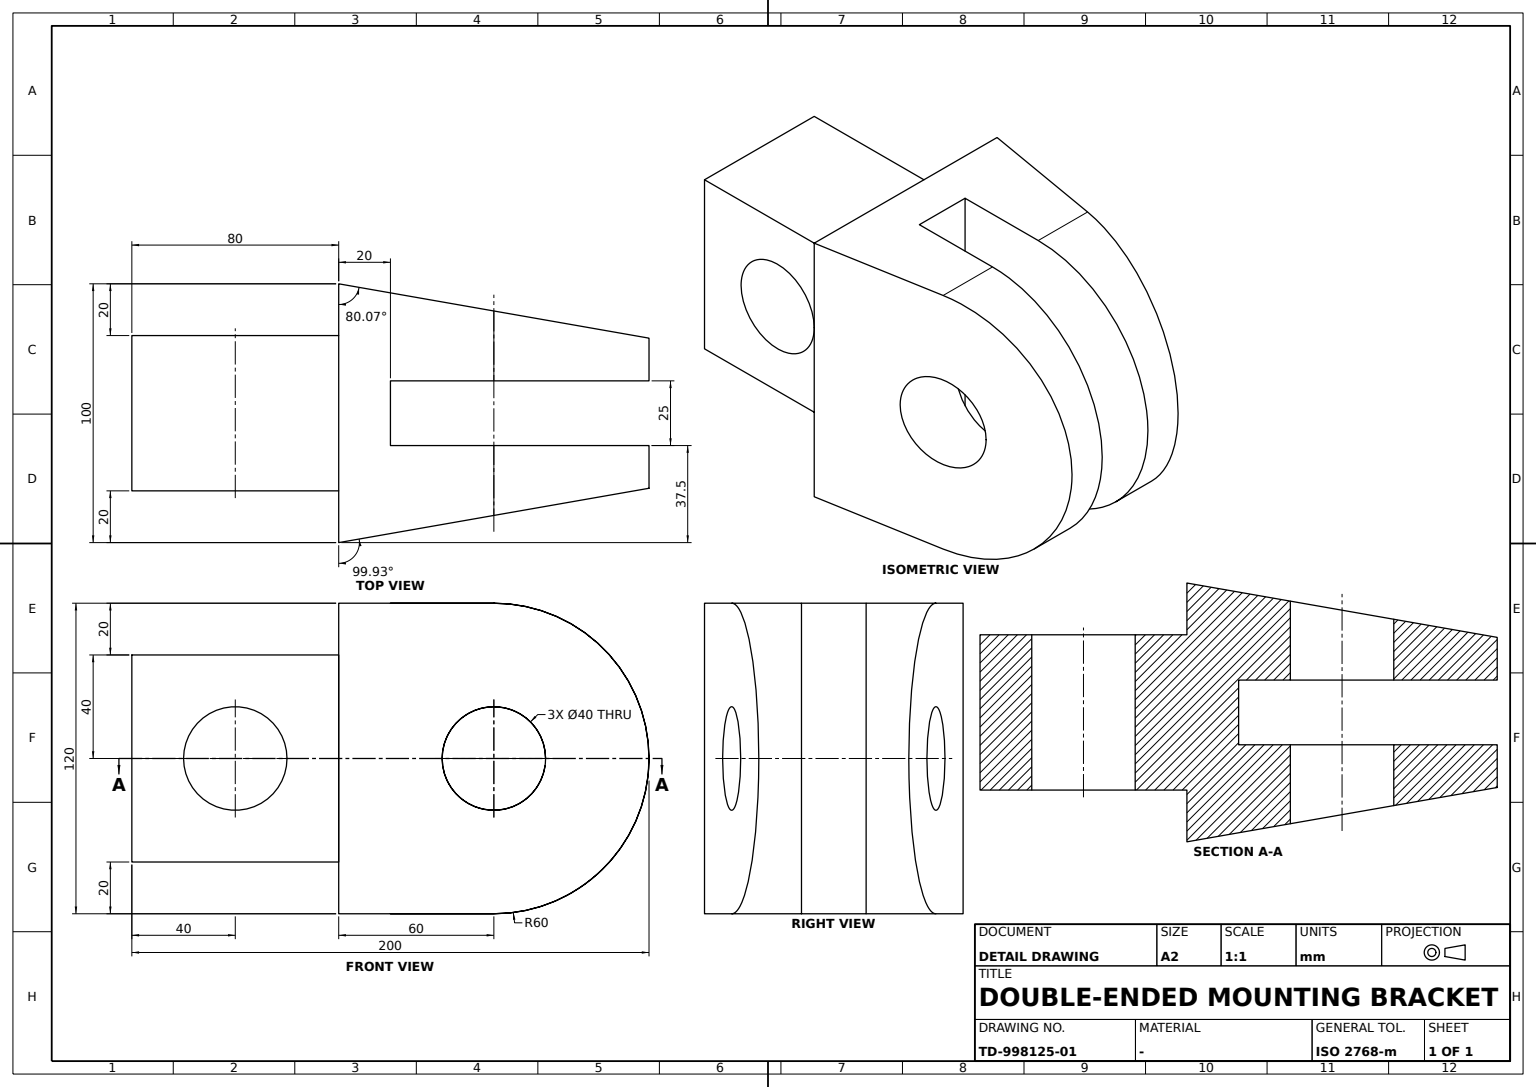
ISO-10303-21;
HEADER;
FILE_DESCRIPTION((''),'2;1');
FILE_NAME('','',(''),(''),'','','');
FILE_SCHEMA(('AUTOMOTIVE_DESIGN'));
ENDSEC;
DATA;
#1=APPLICATION_CONTEXT('');
#2=PRODUCT_CONTEXT('',#1,'mechanical');
#3=PRODUCT('','','',(#2));
#4=PRODUCT_DEFINITION_FORMATION('','',#3);
#5=PRODUCT_DEFINITION_CONTEXT('',#1,'design');
#6=PRODUCT_DEFINITION('','',#4,#5);
#7=PRODUCT_DEFINITION_SHAPE('','',#6);
#8=(LENGTH_UNIT()NAMED_UNIT(*)SI_UNIT(.MILLI.,.METRE.));
#9=(NAMED_UNIT(*)PLANE_ANGLE_UNIT()SI_UNIT($,.RADIAN.));
#10=(NAMED_UNIT(*)SI_UNIT($,.STERADIAN.)SOLID_ANGLE_UNIT());
#11=UNCERTAINTY_MEASURE_WITH_UNIT(LENGTH_MEASURE(1.E-05),#8,'distance_accuracy_value','');
#12=(GEOMETRIC_REPRESENTATION_CONTEXT(3)GLOBAL_UNCERTAINTY_ASSIGNED_CONTEXT((#11))GLOBAL_UNIT_ASSIGNED_CONTEXT((#8,#9,#10))REPRESENTATION_CONTEXT('',''));
#13=CARTESIAN_POINT('',(12.5,-40.,-60.));
#14=VERTEX_POINT('',#13);
#15=CARTESIAN_POINT('',(12.5,0.,-60.));
#16=VERTEX_POINT('',#15);
#17=CARTESIAN_POINT('',(12.5,-20.,-60.));
#18=DIRECTION('',(0.,1.,0.));
#19=VECTOR('',#18,1000.);
#20=LINE('',#17,#19);
#21=EDGE_CURVE('',#14,#16,#20,.T.);
#22=ORIENTED_EDGE('',*,*,#21,.F.);
#23=CARTESIAN_POINT('',(12.5,-40.,60.));
#24=VERTEX_POINT('',#23);
#25=CARTESIAN_POINT('',(12.5,-40.,0.));
#26=DIRECTION('',(0.,0.,-1.));
#27=VECTOR('',#26,1000.);
#28=LINE('',#25,#27);
#29=EDGE_CURVE('',#24,#14,#28,.T.);
#30=ORIENTED_EDGE('',*,*,#29,.F.);
#31=CARTESIAN_POINT('',(12.5,0.,60.));
#32=VERTEX_POINT('',#31);
#33=CARTESIAN_POINT('',(12.5,-20.,60.));
#34=LINE('',#33,#19);
#35=EDGE_CURVE('',#24,#32,#34,.T.);
#36=ORIENTED_EDGE('',*,*,#35,.T.);
#37=CARTESIAN_POINT('',(12.5,60.,0.));
#38=VERTEX_POINT('',#37);
#39=CARTESIAN_POINT('',(12.5,0.,0.));
#40=DIRECTION('',(1.,0.,0.));
#41=DIRECTION('',(0.,-1.,0.));
#42=AXIS2_PLACEMENT_3D('',#39,#40,#41);
#43=CIRCLE('',#42,60.);
#44=EDGE_CURVE('',#38,#32,#43,.T.);
#45=ORIENTED_EDGE('',*,*,#44,.F.);
#46=EDGE_CURVE('',#16,#38,#43,.T.);
#47=ORIENTED_EDGE('',*,*,#46,.F.);
#48=EDGE_LOOP('',(#22,#30,#36,#45,#47));
#49=FACE_OUTER_BOUND('',#48,.T.);
#50=CARTESIAN_POINT('',(12.5,20.,0.));
#51=VERTEX_POINT('',#50);
#52=CARTESIAN_POINT('',(12.5,-20.,0.));
#53=VERTEX_POINT('',#52);
#54=CIRCLE('',#42,20.);
#55=EDGE_CURVE('',#51,#53,#54,.T.);
#56=ORIENTED_EDGE('',*,*,#55,.T.);
#57=EDGE_CURVE('',#53,#51,#54,.T.);
#58=ORIENTED_EDGE('',*,*,#57,.T.);
#59=EDGE_LOOP('',(#56,#58));
#60=FACE_BOUND('',#59,.T.);
#61=CARTESIAN_POINT('',(12.5,77.214676,60.));
#62=AXIS2_PLACEMENT_3D('',#61,#40,#41);
#63=PLANE('',#62);
#64=ADVANCED_FACE('',(#49,#60),#63,.F.);
#65=CARTESIAN_POINT('',(-12.5,20.,0.));
#66=VERTEX_POINT('',#65);
#67=CARTESIAN_POINT('',(-12.5,-20.,0.));
#68=VERTEX_POINT('',#67);
#69=CARTESIAN_POINT('',(-12.5,0.,0.));
#70=DIRECTION('',(-1.,0.,0.));
#71=AXIS2_PLACEMENT_3D('',#69,#70,#18);
#72=CIRCLE('',#71,20.);
#73=EDGE_CURVE('',#66,#68,#72,.T.);
#74=ORIENTED_EDGE('',*,*,#73,.F.);
#75=CARTESIAN_POINT('',(-36.,20.,0.));
#76=VERTEX_POINT('',#75);
#77=CARTESIAN_POINT('',(-0.66,20.,0.));
#78=VECTOR('',#70,1000.);
#79=LINE('',#77,#78);
#80=EDGE_CURVE('',#66,#76,#79,.T.);
#81=ORIENTED_EDGE('',*,*,#80,.T.);
#82=CARTESIAN_POINT('',(-42.999999,-20.,0.));
#83=VERTEX_POINT('',#82);
#84=CARTESIAN_POINT('',(-42.999999,-19.999994,-1.218732));
#85=CARTESIAN_POINT('',(-42.983753,-19.90716,-2.437462));
#86=CARTESIAN_POINT('',(-42.951263,-19.721501,-3.646476));
#87=CARTESIAN_POINT('',(-42.833603,-19.049161,-6.535238));
#88=CARTESIAN_POINT('',(-42.625053,-17.857447,-9.25575));
#89=CARTESIAN_POINT('',(-42.472523,-16.985847,-10.771201));
#90=CARTESIAN_POINT('',(-42.11097,-14.919828,-13.601309));
#91=CARTESIAN_POINT('',(-41.652871,-12.30212,-15.914277));
#92=CARTESIAN_POINT('',(-41.401497,-10.865696,-16.926953));
#93=CARTESIAN_POINT('',(-40.839949,-7.656852,-18.700547));
#94=CARTESIAN_POINT('',(-40.223795,-4.135971,-19.70666));
#95=CARTESIAN_POINT('',(-39.892721,-2.24412,-20.010333));
#96=CARTESIAN_POINT('',(-39.250249,1.427151,-20.157864));
#97=CARTESIAN_POINT('',(-38.618783,5.035523,-19.47528));
#98=CARTESIAN_POINT('',(-38.322943,6.726041,-18.958274));
#99=CARTESIAN_POINT('',(-37.757941,9.954625,-17.566907));
#100=CARTESIAN_POINT('',(-37.257588,12.813783,-15.505126));
#101=CARTESIAN_POINT('',(-37.028803,14.121128,-14.325447));
#102=CARTESIAN_POINT('',(-36.621836,16.446649,-11.710301));
#103=CARTESIAN_POINT('',(-36.32202,18.159888,-8.646962));
#104=CARTESIAN_POINT('',(-36.202412,18.84336,-7.035318));
#105=CARTESIAN_POINT('',(-36.077188,19.558925,-4.653904));
#106=CARTESIAN_POINT('',(-36.01769,19.898913,-2.200641));
#107=CARTESIAN_POINT('',(-36.005897,19.966304,-1.468511));
#108=CARTESIAN_POINT('',(-36.,20.,-0.734255));
#109=B_SPLINE_CURVE_WITH_KNOTS('',5,(#82,#84,#85,#86,#87,#88,#89,#90,#91,#92,#93,#94,#95,#96,#97,#98,#99,#100,#101,#102,#103,#104,#105,#106,#107,#108,#75),.UNSPECIFIED.,.F.,.F.,(6,3,3,3,3,3,3,3,6),(89.533426243,98.151203404,110.460544169,122.915174615,136.537729583,149.11185729,161.567661291,173.874806578,179.066776811),.UNSPECIFIED.);
#110=EDGE_CURVE('',#83,#76,#109,.T.);
#111=ORIENTED_EDGE('',*,*,#110,.F.);
#112=CARTESIAN_POINT('',(-0.66,-20.,0.));
#113=LINE('',#112,#78);
#114=EDGE_CURVE('',#68,#83,#113,.T.);
#115=ORIENTED_EDGE('',*,*,#114,.F.);
#116=EDGE_LOOP('',(#74,#81,#111,#115));
#117=FACE_OUTER_BOUND('',#116,.T.);
#118=CARTESIAN_POINT('',(-0.66,0.,0.));
#119=AXIS2_PLACEMENT_3D('',#118,#70,#18);
#120=CYLINDRICAL_SURFACE('',#119,20.);
#121=ADVANCED_FACE('',(#117),#120,.F.);
#122=CARTESIAN_POINT('',(-50.,-60.,60.));
#123=VERTEX_POINT('',#122);
#124=CARTESIAN_POINT('',(50.,-60.,60.));
#125=VERTEX_POINT('',#124);
#126=CARTESIAN_POINT('',(0.,-60.,60.));
#127=VECTOR('',#40,1000.);
#128=LINE('',#126,#127);
#129=EDGE_CURVE('',#123,#125,#128,.T.);
#130=ORIENTED_EDGE('',*,*,#129,.F.);
#131=CARTESIAN_POINT('',(-50.,-60.,-60.));
#132=VERTEX_POINT('',#131);
#133=CARTESIAN_POINT('',(-50.,-60.,0.));
#134=LINE('',#133,#27);
#135=EDGE_CURVE('',#123,#132,#134,.T.);
#136=ORIENTED_EDGE('',*,*,#135,.T.);
#137=CARTESIAN_POINT('',(50.,-60.,-60.));
#138=VERTEX_POINT('',#137);
#139=CARTESIAN_POINT('',(0.,-60.,-60.));
#140=LINE('',#139,#127);
#141=EDGE_CURVE('',#132,#138,#140,.T.);
#142=ORIENTED_EDGE('',*,*,#141,.T.);
#143=CARTESIAN_POINT('',(50.,-60.,0.));
#144=LINE('',#143,#27);
#145=EDGE_CURVE('',#125,#138,#144,.T.);
#146=ORIENTED_EDGE('',*,*,#145,.F.);
#147=EDGE_LOOP('',(#130,#136,#142,#146));
#148=FACE_OUTER_BOUND('',#147,.T.);
#149=CARTESIAN_POINT('',(30.,-60.,-40.));
#150=VERTEX_POINT('',#149);
#151=CARTESIAN_POINT('',(30.,-60.,40.));
#152=VERTEX_POINT('',#151);
#153=CARTESIAN_POINT('',(30.,-60.,0.));
#154=DIRECTION('',(0.,0.,1.));
#155=VECTOR('',#154,1000.);
#156=LINE('',#153,#155);
#157=EDGE_CURVE('',#150,#152,#156,.T.);
#158=ORIENTED_EDGE('',*,*,#157,.F.);
#159=CARTESIAN_POINT('',(-30.,-60.,-40.));
#160=VERTEX_POINT('',#159);
#161=CARTESIAN_POINT('',(0.,-60.,-40.));
#162=LINE('',#161,#127);
#163=EDGE_CURVE('',#160,#150,#162,.T.);
#164=ORIENTED_EDGE('',*,*,#163,.F.);
#165=CARTESIAN_POINT('',(-30.,-60.,40.));
#166=VERTEX_POINT('',#165);
#167=CARTESIAN_POINT('',(-30.,-60.,0.));
#168=LINE('',#167,#155);
#169=EDGE_CURVE('',#160,#166,#168,.T.);
#170=ORIENTED_EDGE('',*,*,#169,.T.);
#171=CARTESIAN_POINT('',(0.,-60.,40.));
#172=LINE('',#171,#127);
#173=EDGE_CURVE('',#166,#152,#172,.T.);
#174=ORIENTED_EDGE('',*,*,#173,.T.);
#175=EDGE_LOOP('',(#158,#164,#170,#174));
#176=FACE_BOUND('',#175,.T.);
#177=AXIS2_PLACEMENT_3D('',#126,#41,#26);
#178=PLANE('',#177);
#179=ADVANCED_FACE('',(#148,#176),#178,.T.);
#180=CARTESIAN_POINT('',(-30.,-140.,-40.));
#181=VERTEX_POINT('',#180);
#182=CARTESIAN_POINT('',(-30.,-100.,-40.));
#183=LINE('',#182,#19);
#184=EDGE_CURVE('',#181,#160,#183,.T.);
#185=ORIENTED_EDGE('',*,*,#184,.F.);
#186=CARTESIAN_POINT('',(-30.,-140.,40.));
#187=VERTEX_POINT('',#186);
#188=CARTESIAN_POINT('',(-30.,-140.,0.));
#189=LINE('',#188,#27);
#190=EDGE_CURVE('',#187,#181,#189,.T.);
#191=ORIENTED_EDGE('',*,*,#190,.F.);
#192=CARTESIAN_POINT('',(-30.,-100.,40.));
#193=VECTOR('',#41,1000.);
#194=LINE('',#192,#193);
#195=EDGE_CURVE('',#166,#187,#194,.T.);
#196=ORIENTED_EDGE('',*,*,#195,.F.);
#197=ORIENTED_EDGE('',*,*,#169,.F.);
#198=EDGE_LOOP('',(#185,#191,#196,#197));
#199=FACE_OUTER_BOUND('',#198,.T.);
#200=CARTESIAN_POINT('',(-30.,-80.,0.));
#201=VERTEX_POINT('',#200);
#202=CARTESIAN_POINT('',(-30.,-120.,0.));
#203=VERTEX_POINT('',#202);
#204=CARTESIAN_POINT('',(-30.,-100.,0.));
#205=AXIS2_PLACEMENT_3D('',#204,#40,#18);
#206=CIRCLE('',#205,20.);
#207=EDGE_CURVE('',#201,#203,#206,.T.);
#208=ORIENTED_EDGE('',*,*,#207,.T.);
#209=EDGE_CURVE('',#203,#201,#206,.T.);
#210=ORIENTED_EDGE('',*,*,#209,.T.);
#211=EDGE_LOOP('',(#208,#210));
#212=FACE_BOUND('',#211,.T.);
#213=CARTESIAN_POINT('',(-30.,0.,0.));
#214=AXIS2_PLACEMENT_3D('',#213,#40,#18);
#215=PLANE('',#214);
#216=ADVANCED_FACE('',(#199,#212),#215,.F.);
#217=CARTESIAN_POINT('',(30.,-120.,0.));
#218=VERTEX_POINT('',#217);
#219=CARTESIAN_POINT('',(-10.66,-120.,0.));
#220=LINE('',#219,#78);
#221=EDGE_CURVE('',#218,#203,#220,.T.);
#222=ORIENTED_EDGE('',*,*,#221,.F.);
#223=CARTESIAN_POINT('',(30.,-80.,0.));
#224=VERTEX_POINT('',#223);
#225=CARTESIAN_POINT('',(30.,-100.,0.));
#226=AXIS2_PLACEMENT_3D('',#225,#40,#18);
#227=CIRCLE('',#226,20.);
#228=EDGE_CURVE('',#218,#224,#227,.T.);
#229=ORIENTED_EDGE('',*,*,#228,.T.);
#230=CARTESIAN_POINT('',(-10.66,-80.,0.));
#231=LINE('',#230,#78);
#232=EDGE_CURVE('',#224,#201,#231,.T.);
#233=ORIENTED_EDGE('',*,*,#232,.T.);
#234=ORIENTED_EDGE('',*,*,#209,.F.);
#235=EDGE_LOOP('',(#222,#229,#233,#234));
#236=FACE_OUTER_BOUND('',#235,.T.);
#237=CARTESIAN_POINT('',(-10.66,-100.,0.));
#238=AXIS2_PLACEMENT_3D('',#237,#70,#18);
#239=CYLINDRICAL_SURFACE('',#238,20.);
#240=ADVANCED_FACE('',(#236),#239,.F.);
#241=CARTESIAN_POINT('',(30.,-140.,-40.));
#242=VERTEX_POINT('',#241);
#243=CARTESIAN_POINT('',(0.,-140.,-40.));
#244=LINE('',#243,#127);
#245=EDGE_CURVE('',#181,#242,#244,.T.);
#246=ORIENTED_EDGE('',*,*,#245,.F.);
#247=ORIENTED_EDGE('',*,*,#184,.T.);
#248=ORIENTED_EDGE('',*,*,#163,.T.);
#249=CARTESIAN_POINT('',(30.,-100.,-40.));
#250=LINE('',#249,#19);
#251=EDGE_CURVE('',#242,#150,#250,.T.);
#252=ORIENTED_EDGE('',*,*,#251,.F.);
#253=EDGE_LOOP('',(#246,#247,#248,#252));
#254=FACE_OUTER_BOUND('',#253,.T.);
#255=AXIS2_PLACEMENT_3D('',#243,#26,#18);
#256=PLANE('',#255);
#257=ADVANCED_FACE('',(#254),#256,.T.);
#258=ORIENTED_EDGE('',*,*,#73,.T.);
#259=EDGE_CURVE('',#68,#66,#72,.T.);
#260=ORIENTED_EDGE('',*,*,#259,.T.);
#261=EDGE_LOOP('',(#258,#260));
#262=FACE_BOUND('',#261,.T.);
#263=CARTESIAN_POINT('',(-12.5,0.,60.));
#264=VERTEX_POINT('',#263);
#265=CARTESIAN_POINT('',(-12.5,-40.,60.));
#266=VERTEX_POINT('',#265);
#267=CARTESIAN_POINT('',(-12.5,-20.,60.));
#268=LINE('',#267,#193);
#269=EDGE_CURVE('',#264,#266,#268,.T.);
#270=ORIENTED_EDGE('',*,*,#269,.T.);
#271=CARTESIAN_POINT('',(-12.5,-40.,-60.));
#272=VERTEX_POINT('',#271);
#273=CARTESIAN_POINT('',(-12.5,-40.,0.));
#274=LINE('',#273,#27);
#275=EDGE_CURVE('',#266,#272,#274,.T.);
#276=ORIENTED_EDGE('',*,*,#275,.T.);
#277=CARTESIAN_POINT('',(-12.5,0.,-60.));
#278=VERTEX_POINT('',#277);
#279=CARTESIAN_POINT('',(-12.5,-20.,-60.));
#280=LINE('',#279,#19);
#281=EDGE_CURVE('',#272,#278,#280,.T.);
#282=ORIENTED_EDGE('',*,*,#281,.T.);
#283=CARTESIAN_POINT('',(-12.5,60.,0.));
#284=VERTEX_POINT('',#283);
#285=CIRCLE('',#71,60.);
#286=EDGE_CURVE('',#284,#278,#285,.T.);
#287=ORIENTED_EDGE('',*,*,#286,.F.);
#288=EDGE_CURVE('',#264,#284,#285,.T.);
#289=ORIENTED_EDGE('',*,*,#288,.F.);
#290=EDGE_LOOP('',(#270,#276,#282,#287,#289));
#291=FACE_OUTER_BOUND('',#290,.T.);
#292=AXIS2_PLACEMENT_3D('',#265,#70,#18);
#293=PLANE('',#292);
#294=ADVANCED_FACE('',(#262,#291),#293,.F.);
#295=CARTESIAN_POINT('',(-39.5,0.,60.));
#296=VERTEX_POINT('',#295);
#297=CARTESIAN_POINT('',(-44.75,-30.,60.));
#298=DIRECTION('',(0.172380332,0.985030467,0.));
#299=VECTOR('',#298,1000.);
#300=LINE('',#297,#299);
#301=EDGE_CURVE('',#123,#296,#300,.T.);
#302=ORIENTED_EDGE('',*,*,#301,.T.);
#303=CARTESIAN_POINT('',(-29.,60.,0.));
#304=VERTEX_POINT('',#303);
#305=CARTESIAN_POINT('',(-29.,59.999999,3.493208));
#306=CARTESIAN_POINT('',(-29.044489,59.745776,6.986413));
#307=CARTESIAN_POINT('',(-29.133467,59.237334,10.454186));
#308=CARTESIAN_POINT('',(-29.437777,57.498419,18.28685));
#309=CARTESIAN_POINT('',(-29.964905,54.486256,25.726527));
#310=CARTESIAN_POINT('',(-30.329947,52.400304,29.744072));
#311=CARTESIAN_POINT('',(-31.190529,47.482693,37.368993));
#312=CARTESIAN_POINT('',(-32.281743,41.24718,43.926827));
#313=CARTESIAN_POINT('',(-32.882146,37.816307,46.911581));
#314=CARTESIAN_POINT('',(-34.178522,30.408443,52.219117));
#315=CARTESIAN_POINT('',(-35.622408,22.157671,56.037695));
#316=CARTESIAN_POINT('',(-36.376884,17.846376,57.555296));
#317=CARTESIAN_POINT('',(-37.457426,11.671853,59.090372));
#318=CARTESIAN_POINT('',(-38.559098,5.376584,59.799011));
#319=CARTESIAN_POINT('',(-38.872354,3.586547,59.933004));
#320=CARTESIAN_POINT('',(-39.186177,1.793273,60.));
#321=B_SPLINE_CURVE_WITH_KNOTS('',5,(#303,#305,#306,#307,#308,#309,#310,#311,#312,#313,#314,#315,#316,#317,#318,#319,#320,#295),.UNSPECIFIED.,.F.,.F.,(6,3,3,3,3,6),(134.300512617,159.001235304,190.921926195,223.164321771,255.72815621,268.601217848),.UNSPECIFIED.);
#322=EDGE_CURVE('',#304,#296,#321,.T.);
#323=ORIENTED_EDGE('',*,*,#322,.F.);
#324=CARTESIAN_POINT('',(-39.5,0.,-60.));
#325=VERTEX_POINT('',#324);
#326=CARTESIAN_POINT('',(-38.656215,4.821627,-60.));
#327=CARTESIAN_POINT('',(-37.81243,9.643254,-59.515665));
#328=CARTESIAN_POINT('',(-36.979612,14.402219,-58.546932));
#329=CARTESIAN_POINT('',(-35.410917,23.36619,-55.757651));
#330=CARTESIAN_POINT('',(-33.963827,31.635272,-51.284427));
#331=CARTESIAN_POINT('',(-33.30152,35.419884,-48.748672));
#332=CARTESIAN_POINT('',(-32.073505,42.437117,-43.014944));
#333=CARTESIAN_POINT('',(-31.051476,48.277283,-36.053804));
#334=CARTESIAN_POINT('',(-30.600946,50.851738,-32.323259));
#335=CARTESIAN_POINT('',(-29.829797,55.258303,-24.440363));
#336=CARTESIAN_POINT('',(-29.327494,58.128606,-15.858342));
#337=CARTESIAN_POINT('',(-29.148027,59.154134,-11.457178));
#338=CARTESIAN_POINT('',(-29.029953,59.828838,-6.487634));
#339=CARTESIAN_POINT('',(-29.00272,59.98446,-1.495848));
#340=CARTESIAN_POINT('',(-29.000907,59.99482,-0.997281));
#341=CARTESIAN_POINT('',(-29.,60.,-0.498641));
#342=B_SPLINE_CURVE_WITH_KNOTS('',5,(#324,#326,#327,#328,#329,#330,#331,#332,#333,#334,#335,#336,#337,#338,#339,#340,#341,#303),.UNSPECIFIED.,.F.,.F.,(6,3,3,3,3,6),(0.,34.612181975,66.971381031,98.987544351,130.774589311,134.300512617),.UNSPECIFIED.);
#343=EDGE_CURVE('',#325,#304,#342,.T.);
#344=ORIENTED_EDGE('',*,*,#343,.F.);
#345=CARTESIAN_POINT('',(-44.75,-30.,-60.));
#346=LINE('',#345,#299);
#347=EDGE_CURVE('',#132,#325,#346,.T.);
#348=ORIENTED_EDGE('',*,*,#347,.F.);
#349=ORIENTED_EDGE('',*,*,#135,.F.);
#350=EDGE_LOOP('',(#302,#323,#344,#348,#349));
#351=FACE_OUTER_BOUND('',#350,.T.);
#352=CARTESIAN_POINT('',(-36.,20.,1.586513));
#353=CARTESIAN_POINT('',(-36.02753,19.842686,3.173026));
#354=CARTESIAN_POINT('',(-36.082593,19.528037,4.738084));
#355=CARTESIAN_POINT('',(-36.254283,18.546952,7.934391));
#356=CARTESIAN_POINT('',(-36.536928,16.931839,10.857254));
#357=CARTESIAN_POINT('',(-36.713368,15.923613,12.287572));
#358=CARTESIAN_POINT('',(-37.119385,13.603512,14.918356));
#359=CARTESIAN_POINT('',(-37.61339,10.780627,16.982216));
#360=CARTESIAN_POINT('',(-37.880409,9.254806,17.859077));
#361=CARTESIAN_POINT('',(-38.444945,6.028886,19.269994));
#362=CARTESIAN_POINT('',(-39.04843,2.580399,19.949652));
#363=CARTESIAN_POINT('',(-39.356547,0.819732,20.099037));
#364=CARTESIAN_POINT('',(-39.972982,-2.702753,20.010155));
#365=CARTESIAN_POINT('',(-40.571943,-6.125387,19.160355));
#366=CARTESIAN_POINT('',(-40.86214,-7.783658,18.549097));
#367=CARTESIAN_POINT('',(-41.41224,-10.927083,16.978896));
#368=CARTESIAN_POINT('',(-41.891335,-13.664772,14.760393));
#369=CARTESIAN_POINT('',(-42.108005,-14.902888,13.510069));
#370=CARTESIAN_POINT('',(-42.488437,-17.07678,10.770194));
#371=CARTESIAN_POINT('',(-42.757594,-18.614821,7.618052));
#372=CARTESIAN_POINT('',(-42.861176,-19.206718,5.971833));
#373=CARTESIAN_POINT('',(-42.953721,-19.73555,3.773232));
#374=CARTESIAN_POINT('',(-42.991423,-19.950986,1.533124));
#375=CARTESIAN_POINT('',(-42.997141,-19.983661,1.02256));
#376=CARTESIAN_POINT('',(-43.,-19.999998,0.51128));
#377=B_SPLINE_CURVE_WITH_KNOTS('',5,(#75,#352,#353,#354,#355,#356,#357,#358,#359,#360,#361,#362,#363,#364,#365,#366,#367,#368,#369,#370,#371,#372,#373,#374,#375,#376,#82),.UNSPECIFIED.,.F.,.F.,(6,3,3,3,3,3,3,3,6),(0.,11.218341231,23.555732288,36.042726258,48.626253532,61.190537994,73.626504777,85.918119796,89.533426243),.UNSPECIFIED.);
#378=EDGE_CURVE('',#76,#83,#377,.T.);
#379=ORIENTED_EDGE('',*,*,#378,.T.);
#380=ORIENTED_EDGE('',*,*,#110,.T.);
#381=EDGE_LOOP('',(#379,#380));
#382=FACE_BOUND('',#381,.T.);
#383=CARTESIAN_POINT('',(-29.,60.,60.));
#384=DIRECTION('',(0.985030467,-0.172380332,0.));
#385=DIRECTION('',(-0.172380332,-0.985030467,0.));
#386=AXIS2_PLACEMENT_3D('',#383,#384,#385);
#387=PLANE('',#386);
#388=ADVANCED_FACE('',(#351,#382),#387,.F.);
#389=ORIENTED_EDGE('',*,*,#245,.T.);
#390=CARTESIAN_POINT('',(30.,-140.,40.));
#391=VERTEX_POINT('',#390);
#392=CARTESIAN_POINT('',(30.,-140.,0.));
#393=LINE('',#392,#27);
#394=EDGE_CURVE('',#391,#242,#393,.T.);
#395=ORIENTED_EDGE('',*,*,#394,.F.);
#396=CARTESIAN_POINT('',(0.,-140.,40.));
#397=LINE('',#396,#127);
#398=EDGE_CURVE('',#187,#391,#397,.T.);
#399=ORIENTED_EDGE('',*,*,#398,.F.);
#400=ORIENTED_EDGE('',*,*,#190,.T.);
#401=EDGE_LOOP('',(#389,#395,#399,#400));
#402=FACE_OUTER_BOUND('',#401,.T.);
#403=AXIS2_PLACEMENT_3D('',#396,#41,#26);
#404=PLANE('',#403);
#405=ADVANCED_FACE('',(#402),#404,.T.);
#406=ORIENTED_EDGE('',*,*,#80,.F.);
#407=ORIENTED_EDGE('',*,*,#259,.F.);
#408=ORIENTED_EDGE('',*,*,#114,.T.);
#409=ORIENTED_EDGE('',*,*,#378,.F.);
#410=EDGE_LOOP('',(#406,#407,#408,#409));
#411=FACE_OUTER_BOUND('',#410,.T.);
#412=ADVANCED_FACE('',(#411),#120,.F.);
#413=CARTESIAN_POINT('',(0.,-40.,-60.));
#414=LINE('',#413,#127);
#415=EDGE_CURVE('',#272,#14,#414,.T.);
#416=ORIENTED_EDGE('',*,*,#415,.F.);
#417=ORIENTED_EDGE('',*,*,#275,.F.);
#418=CARTESIAN_POINT('',(0.,-40.,60.));
#419=LINE('',#418,#127);
#420=EDGE_CURVE('',#266,#24,#419,.T.);
#421=ORIENTED_EDGE('',*,*,#420,.T.);
#422=ORIENTED_EDGE('',*,*,#29,.T.);
#423=EDGE_LOOP('',(#416,#417,#421,#422));
#424=FACE_OUTER_BOUND('',#423,.T.);
#425=AXIS2_PLACEMENT_3D('',#265,#18,#40);
#426=PLANE('',#425);
#427=ADVANCED_FACE('',(#424),#426,.T.);
#428=CARTESIAN_POINT('',(0.,0.,60.));
#429=LINE('',#428,#127);
#430=EDGE_CURVE('',#296,#264,#429,.T.);
#431=ORIENTED_EDGE('',*,*,#430,.T.);
#432=ORIENTED_EDGE('',*,*,#288,.T.);
#433=CARTESIAN_POINT('',(0.,60.,0.));
#434=LINE('',#433,#78);
#435=EDGE_CURVE('',#284,#304,#434,.T.);
#436=ORIENTED_EDGE('',*,*,#435,.T.);
#437=ORIENTED_EDGE('',*,*,#322,.T.);
#438=EDGE_LOOP('',(#431,#432,#436,#437));
#439=FACE_OUTER_BOUND('',#438,.T.);
#440=CARTESIAN_POINT('',(0.,0.,0.));
#441=AXIS2_PLACEMENT_3D('',#440,#70,#18);
#442=CYLINDRICAL_SURFACE('',#441,60.);
#443=ADVANCED_FACE('',(#439),#442,.T.);
#444=ORIENTED_EDGE('',*,*,#269,.F.);
#445=ORIENTED_EDGE('',*,*,#430,.F.);
#446=ORIENTED_EDGE('',*,*,#301,.F.);
#447=ORIENTED_EDGE('',*,*,#129,.T.);
#448=CARTESIAN_POINT('',(39.5,0.,60.));
#449=VERTEX_POINT('',#448);
#450=CARTESIAN_POINT('',(44.75,-30.,60.));
#451=DIRECTION('',(0.172380332,-0.985030467,0.));
#452=VECTOR('',#451,1000.);
#453=LINE('',#450,#452);
#454=EDGE_CURVE('',#449,#125,#453,.T.);
#455=ORIENTED_EDGE('',*,*,#454,.F.);
#456=EDGE_CURVE('',#32,#449,#429,.T.);
#457=ORIENTED_EDGE('',*,*,#456,.F.);
#458=ORIENTED_EDGE('',*,*,#35,.F.);
#459=ORIENTED_EDGE('',*,*,#420,.F.);
#460=EDGE_LOOP('',(#444,#445,#446,#447,#455,#457,#458,#459));
#461=FACE_OUTER_BOUND('',#460,.T.);
#462=AXIS2_PLACEMENT_3D('',#126,#26,#18);
#463=PLANE('',#462);
#464=ADVANCED_FACE('',(#461),#463,.F.);
#465=ORIENTED_EDGE('',*,*,#415,.T.);
#466=ORIENTED_EDGE('',*,*,#21,.T.);
#467=CARTESIAN_POINT('',(39.5,0.,-60.));
#468=VERTEX_POINT('',#467);
#469=CARTESIAN_POINT('',(0.,0.,-60.));
#470=LINE('',#469,#127);
#471=EDGE_CURVE('',#16,#468,#470,.T.);
#472=ORIENTED_EDGE('',*,*,#471,.T.);
#473=CARTESIAN_POINT('',(44.75,-30.,-60.));
#474=DIRECTION('',(-0.172380332,0.985030467,0.));
#475=VECTOR('',#474,1000.);
#476=LINE('',#473,#475);
#477=EDGE_CURVE('',#138,#468,#476,.T.);
#478=ORIENTED_EDGE('',*,*,#477,.F.);
#479=ORIENTED_EDGE('',*,*,#141,.F.);
#480=ORIENTED_EDGE('',*,*,#347,.T.);
#481=EDGE_CURVE('',#325,#278,#470,.T.);
#482=ORIENTED_EDGE('',*,*,#481,.T.);
#483=ORIENTED_EDGE('',*,*,#281,.F.);
#484=EDGE_LOOP('',(#465,#466,#472,#478,#479,#480,#482,#483));
#485=FACE_OUTER_BOUND('',#484,.T.);
#486=AXIS2_PLACEMENT_3D('',#139,#26,#18);
#487=PLANE('',#486);
#488=ADVANCED_FACE('',(#485),#487,.T.);
#489=ORIENTED_EDGE('',*,*,#481,.F.);
#490=ORIENTED_EDGE('',*,*,#343,.T.);
#491=ORIENTED_EDGE('',*,*,#435,.F.);
#492=ORIENTED_EDGE('',*,*,#286,.T.);
#493=EDGE_LOOP('',(#489,#490,#491,#492));
#494=FACE_OUTER_BOUND('',#493,.T.);
#495=ADVANCED_FACE('',(#494),#442,.T.);
#496=CARTESIAN_POINT('',(30.,-100.,40.));
#497=LINE('',#496,#193);
#498=EDGE_CURVE('',#152,#391,#497,.T.);
#499=ORIENTED_EDGE('',*,*,#498,.F.);
#500=ORIENTED_EDGE('',*,*,#173,.F.);
#501=ORIENTED_EDGE('',*,*,#195,.T.);
#502=ORIENTED_EDGE('',*,*,#398,.T.);
#503=EDGE_LOOP('',(#499,#500,#501,#502));
#504=FACE_OUTER_BOUND('',#503,.T.);
#505=AXIS2_PLACEMENT_3D('',#396,#26,#18);
#506=PLANE('',#505);
#507=ADVANCED_FACE('',(#504),#506,.F.);
#508=ORIENTED_EDGE('',*,*,#55,.F.);
#509=CARTESIAN_POINT('',(36.,20.,0.));
#510=VERTEX_POINT('',#509);
#511=EDGE_CURVE('',#510,#51,#79,.T.);
#512=ORIENTED_EDGE('',*,*,#511,.F.);
#513=CARTESIAN_POINT('',(42.999999,-20.,0.));
#514=VERTEX_POINT('',#513);
#515=CARTESIAN_POINT('',(36.,20.,1.586513));
#516=CARTESIAN_POINT('',(36.02753,19.842686,3.173026));
#517=CARTESIAN_POINT('',(36.082593,19.528037,4.738084));
#518=CARTESIAN_POINT('',(36.254283,18.546952,7.934391));
#519=CARTESIAN_POINT('',(36.536928,16.931839,10.857254));
#520=CARTESIAN_POINT('',(36.713368,15.923613,12.287572));
#521=CARTESIAN_POINT('',(37.119385,13.603512,14.918356));
#522=CARTESIAN_POINT('',(37.61339,10.780627,16.982216));
#523=CARTESIAN_POINT('',(37.880409,9.254806,17.859077));
#524=CARTESIAN_POINT('',(38.444945,6.028886,19.269994));
#525=CARTESIAN_POINT('',(39.04843,2.580399,19.949652));
#526=CARTESIAN_POINT('',(39.356547,0.819732,20.099037));
#527=CARTESIAN_POINT('',(39.972982,-2.702753,20.010155));
#528=CARTESIAN_POINT('',(40.571943,-6.125387,19.160355));
#529=CARTESIAN_POINT('',(40.86214,-7.783658,18.549097));
#530=CARTESIAN_POINT('',(41.41224,-10.927083,16.978896));
#531=CARTESIAN_POINT('',(41.891335,-13.664772,14.760393));
#532=CARTESIAN_POINT('',(42.108005,-14.902888,13.510069));
#533=CARTESIAN_POINT('',(42.488437,-17.07678,10.770194));
#534=CARTESIAN_POINT('',(42.757594,-18.614821,7.618052));
#535=CARTESIAN_POINT('',(42.861176,-19.206718,5.971833));
#536=CARTESIAN_POINT('',(42.953721,-19.73555,3.773232));
#537=CARTESIAN_POINT('',(42.991423,-19.950986,1.533124));
#538=CARTESIAN_POINT('',(42.997141,-19.983661,1.02256));
#539=CARTESIAN_POINT('',(43.,-19.999998,0.51128));
#540=B_SPLINE_CURVE_WITH_KNOTS('',5,(#509,#515,#516,#517,#518,#519,#520,#521,#522,#523,#524,#525,#526,#527,#528,#529,#530,#531,#532,#533,#534,#535,#536,#537,#538,#539,#513),.UNSPECIFIED.,.F.,.F.,(6,3,3,3,3,3,3,3,6),(0.,11.218341231,23.555732288,36.042726258,48.626253532,61.190537993,73.626504777,85.918119795,89.533426242),.UNSPECIFIED.);
#541=EDGE_CURVE('',#510,#514,#540,.T.);
#542=ORIENTED_EDGE('',*,*,#541,.T.);
#543=EDGE_CURVE('',#514,#53,#113,.T.);
#544=ORIENTED_EDGE('',*,*,#543,.T.);
#545=EDGE_LOOP('',(#508,#512,#542,#544));
#546=FACE_OUTER_BOUND('',#545,.T.);
#547=ADVANCED_FACE('',(#546),#120,.F.);
#548=ORIENTED_EDGE('',*,*,#221,.T.);
#549=ORIENTED_EDGE('',*,*,#207,.F.);
#550=ORIENTED_EDGE('',*,*,#232,.F.);
#551=EDGE_CURVE('',#224,#218,#227,.T.);
#552=ORIENTED_EDGE('',*,*,#551,.T.);
#553=EDGE_LOOP('',(#548,#549,#550,#552));
#554=FACE_OUTER_BOUND('',#553,.T.);
#555=ADVANCED_FACE('',(#554),#239,.F.);
#556=ORIENTED_EDGE('',*,*,#498,.T.);
#557=ORIENTED_EDGE('',*,*,#394,.T.);
#558=ORIENTED_EDGE('',*,*,#251,.T.);
#559=ORIENTED_EDGE('',*,*,#157,.T.);
#560=EDGE_LOOP('',(#556,#557,#558,#559));
#561=FACE_OUTER_BOUND('',#560,.T.);
#562=ORIENTED_EDGE('',*,*,#551,.F.);
#563=ORIENTED_EDGE('',*,*,#228,.F.);
#564=EDGE_LOOP('',(#562,#563));
#565=FACE_BOUND('',#564,.T.);
#566=CARTESIAN_POINT('',(30.,0.,0.));
#567=AXIS2_PLACEMENT_3D('',#566,#40,#18);
#568=PLANE('',#567);
#569=ADVANCED_FACE('',(#561,#565),#568,.T.);
#570=ORIENTED_EDGE('',*,*,#57,.F.);
#571=ORIENTED_EDGE('',*,*,#543,.F.);
#572=CARTESIAN_POINT('',(42.999999,-19.999994,-1.218732));
#573=CARTESIAN_POINT('',(42.983753,-19.90716,-2.437462));
#574=CARTESIAN_POINT('',(42.951263,-19.721501,-3.646476));
#575=CARTESIAN_POINT('',(42.833603,-19.049161,-6.535238));
#576=CARTESIAN_POINT('',(42.625053,-17.857447,-9.25575));
#577=CARTESIAN_POINT('',(42.472523,-16.985847,-10.771201));
#578=CARTESIAN_POINT('',(42.11097,-14.919828,-13.601309));
#579=CARTESIAN_POINT('',(41.652871,-12.30212,-15.914277));
#580=CARTESIAN_POINT('',(41.401497,-10.865696,-16.926953));
#581=CARTESIAN_POINT('',(40.839949,-7.656852,-18.700547));
#582=CARTESIAN_POINT('',(40.223795,-4.135971,-19.70666));
#583=CARTESIAN_POINT('',(39.892721,-2.24412,-20.010333));
#584=CARTESIAN_POINT('',(39.250249,1.427151,-20.157864));
#585=CARTESIAN_POINT('',(38.618783,5.035523,-19.47528));
#586=CARTESIAN_POINT('',(38.322943,6.726041,-18.958274));
#587=CARTESIAN_POINT('',(37.757941,9.954625,-17.566907));
#588=CARTESIAN_POINT('',(37.257588,12.813783,-15.505126));
#589=CARTESIAN_POINT('',(37.028803,14.121128,-14.325447));
#590=CARTESIAN_POINT('',(36.621836,16.446649,-11.710301));
#591=CARTESIAN_POINT('',(36.32202,18.159888,-8.646962));
#592=CARTESIAN_POINT('',(36.202412,18.84336,-7.035318));
#593=CARTESIAN_POINT('',(36.077188,19.558925,-4.653904));
#594=CARTESIAN_POINT('',(36.01769,19.898913,-2.200641));
#595=CARTESIAN_POINT('',(36.005897,19.966304,-1.468511));
#596=CARTESIAN_POINT('',(36.,20.,-0.734255));
#597=B_SPLINE_CURVE_WITH_KNOTS('',5,(#513,#572,#573,#574,#575,#576,#577,#578,#579,#580,#581,#582,#583,#584,#585,#586,#587,#588,#589,#590,#591,#592,#593,#594,#595,#596,#509),.UNSPECIFIED.,.F.,.F.,(6,3,3,3,3,3,3,3,6),(89.533426242,98.151203404,110.460544169,122.915174614,136.537729581,149.111857288,161.567661288,173.874806576,179.066776808),.UNSPECIFIED.);
#598=EDGE_CURVE('',#514,#510,#597,.T.);
#599=ORIENTED_EDGE('',*,*,#598,.T.);
#600=ORIENTED_EDGE('',*,*,#511,.T.);
#601=EDGE_LOOP('',(#570,#571,#599,#600));
#602=FACE_OUTER_BOUND('',#601,.T.);
#603=ADVANCED_FACE('',(#602),#120,.F.);
#604=ORIENTED_EDGE('',*,*,#598,.F.);
#605=ORIENTED_EDGE('',*,*,#541,.F.);
#606=EDGE_LOOP('',(#604,#605));
#607=FACE_BOUND('',#606,.T.);
#608=ORIENTED_EDGE('',*,*,#145,.T.);
#609=ORIENTED_EDGE('',*,*,#477,.T.);
#610=CARTESIAN_POINT('',(29.,60.,0.));
#611=VERTEX_POINT('',#610);
#612=CARTESIAN_POINT('',(38.656215,4.821627,-60.));
#613=CARTESIAN_POINT('',(37.81243,9.643254,-59.515665));
#614=CARTESIAN_POINT('',(36.979612,14.402219,-58.546932));
#615=CARTESIAN_POINT('',(35.410917,23.36619,-55.757651));
#616=CARTESIAN_POINT('',(33.963827,31.635272,-51.284427));
#617=CARTESIAN_POINT('',(33.30152,35.419884,-48.748672));
#618=CARTESIAN_POINT('',(32.073505,42.437117,-43.014944));
#619=CARTESIAN_POINT('',(31.051476,48.277283,-36.053804));
#620=CARTESIAN_POINT('',(30.600946,50.851738,-32.323259));
#621=CARTESIAN_POINT('',(29.829797,55.258303,-24.440363));
#622=CARTESIAN_POINT('',(29.327494,58.128606,-15.858342));
#623=CARTESIAN_POINT('',(29.148027,59.154134,-11.457178));
#624=CARTESIAN_POINT('',(29.029953,59.828838,-6.487634));
#625=CARTESIAN_POINT('',(29.00272,59.98446,-1.495848));
#626=CARTESIAN_POINT('',(29.000907,59.99482,-0.997281));
#627=CARTESIAN_POINT('',(29.,60.,-0.498641));
#628=B_SPLINE_CURVE_WITH_KNOTS('',5,(#467,#612,#613,#614,#615,#616,#617,#618,#619,#620,#621,#622,#623,#624,#625,#626,#627,#610),.UNSPECIFIED.,.F.,.F.,(6,3,3,3,3,6),(0.,34.612181975,66.971381031,98.987544351,130.774589312,134.300512617),.UNSPECIFIED.);
#629=EDGE_CURVE('',#468,#611,#628,.T.);
#630=ORIENTED_EDGE('',*,*,#629,.T.);
#631=CARTESIAN_POINT('',(29.,59.999999,3.493208));
#632=CARTESIAN_POINT('',(29.044489,59.745776,6.986413));
#633=CARTESIAN_POINT('',(29.133467,59.237334,10.454186));
#634=CARTESIAN_POINT('',(29.437777,57.498419,18.28685));
#635=CARTESIAN_POINT('',(29.964905,54.486256,25.726527));
#636=CARTESIAN_POINT('',(30.329947,52.400304,29.744072));
#637=CARTESIAN_POINT('',(31.190529,47.482693,37.368993));
#638=CARTESIAN_POINT('',(32.281743,41.24718,43.926827));
#639=CARTESIAN_POINT('',(32.882146,37.816307,46.911581));
#640=CARTESIAN_POINT('',(34.178522,30.408443,52.219117));
#641=CARTESIAN_POINT('',(35.622408,22.157671,56.037695));
#642=CARTESIAN_POINT('',(36.376884,17.846376,57.555296));
#643=CARTESIAN_POINT('',(37.457426,11.671853,59.090372));
#644=CARTESIAN_POINT('',(38.559098,5.376584,59.799011));
#645=CARTESIAN_POINT('',(38.872354,3.586547,59.933004));
#646=CARTESIAN_POINT('',(39.186177,1.793273,60.));
#647=B_SPLINE_CURVE_WITH_KNOTS('',5,(#610,#631,#632,#633,#634,#635,#636,#637,#638,#639,#640,#641,#642,#643,#644,#645,#646,#448),.UNSPECIFIED.,.F.,.F.,(6,3,3,3,3,6),(134.300512617,159.001235305,190.921926195,223.164321772,255.72815621,268.601217848),.UNSPECIFIED.);
#648=EDGE_CURVE('',#611,#449,#647,.T.);
#649=ORIENTED_EDGE('',*,*,#648,.T.);
#650=ORIENTED_EDGE('',*,*,#454,.T.);
#651=EDGE_LOOP('',(#608,#609,#630,#649,#650));
#652=FACE_OUTER_BOUND('',#651,.T.);
#653=CARTESIAN_POINT('',(29.,60.,60.));
#654=DIRECTION('',(0.985030467,0.172380332,0.));
#655=AXIS2_PLACEMENT_3D('',#653,#654,#451);
#656=PLANE('',#655);
#657=ADVANCED_FACE('',(#607,#652),#656,.T.);
#658=EDGE_CURVE('',#611,#38,#434,.T.);
#659=ORIENTED_EDGE('',*,*,#658,.T.);
#660=ORIENTED_EDGE('',*,*,#44,.T.);
#661=ORIENTED_EDGE('',*,*,#456,.T.);
#662=ORIENTED_EDGE('',*,*,#648,.F.);
#663=EDGE_LOOP('',(#659,#660,#661,#662));
#664=FACE_OUTER_BOUND('',#663,.T.);
#665=ADVANCED_FACE('',(#664),#442,.T.);
#666=ORIENTED_EDGE('',*,*,#658,.F.);
#667=ORIENTED_EDGE('',*,*,#629,.F.);
#668=ORIENTED_EDGE('',*,*,#471,.F.);
#669=ORIENTED_EDGE('',*,*,#46,.T.);
#670=EDGE_LOOP('',(#666,#667,#668,#669));
#671=FACE_OUTER_BOUND('',#670,.T.);
#672=ADVANCED_FACE('',(#671),#442,.T.);
#673=CLOSED_SHELL('',(#64,#121,#179,#216,#240,#257,#294,#388,#405,#412,#427,#443,#464,#488,#495,#507,#547,#555,#569,#603,#657,#665,#672));
#674=MANIFOLD_SOLID_BREP('',#673);
#675=ADVANCED_BREP_SHAPE_REPRESENTATION('',(#674),#12);
#676=SHAPE_DEFINITION_REPRESENTATION(#7,#675);
ENDSEC;
END-ISO-10303-21;
